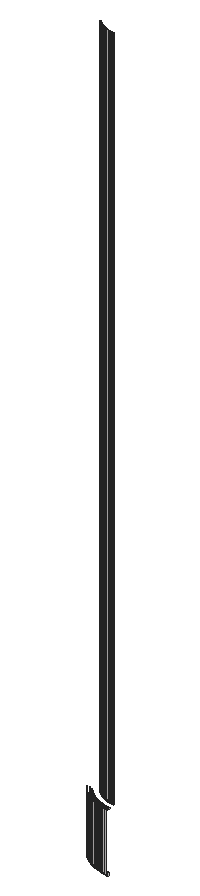
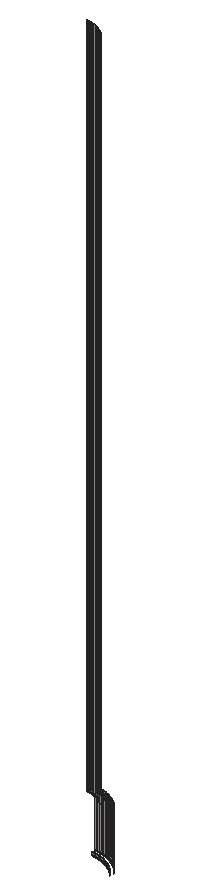
# SketchUp Ruby script. Lengths in inches.
U = 1.inch
M = Sketchup.active_model
def pt(a) = Geom::Point3d.new(a.map { |v| v * U })
def face(e, loops, mat)
  f = e.add_face(loops[0].map { |a| pt(a) })
  loops[1..].each { |l| e.add_face(l.map { |a| pt(a) }).erase! }
  f.material = f.back_material = mat if mat
  f
end
# faces: each face lists its corners as indices into pts; further lists are holes
def faces(e, pts, list, mat = nil) = list.each { |f| face(e, (f[0].is_a?(Array) ? f : [f]).map { |l| l.map { |i| pts[i] } }, mat) }
# xy, xz, yz: faces in a plane at the given z, y or x. An outline is a flat list of corners, or four numbers for a rectangle; further outlines are holes
def ring(l) = l.size == 4 ? [[l[0], l[1]], [l[2], l[1]], [l[2], l[3]], [l[0], l[3]]] : l.each_slice(2).to_a
def flat(e, list, mat, &to3) = list.each { |f| face(e, (f[0].is_a?(Array) ? f : [f]).map { |l| ring(l).map { |u, v| to3.(u, v) } }, mat) }
def xy(e, z, list, mat = nil) = flat(e, list, mat) { |x, y| [x, y, z] }
def xz(e, y, list, mat = nil) = flat(e, list, mat) { |x, z| [x, y, z] }
def yz(e, x, list, mat = nil) = flat(e, list, mat) { |y, z| [x, y, z] }
def lines(e, pts, list) = list.each { |a, b| e.add_line(pt(pts[a]), pt(pts[b])) }
# prism: a flat outline (further loops are holes) pulled along v
def prism(e, loops, v, mat = nil)
  f = face(e, loops, mat); d = Geom::Vector3d.new(v.map { |x| x * U })
  f.pushpull(f.normal.samedirection?(d) ? d.length : -d.length)
end
def box(e, o, s, mat = nil) = prism(e, [[o, [o[0] + s[0], o[1], o[2]], [o[0] + s[0], o[1] + s[1], o[2]], [o[0], o[1] + s[1], o[2]]]], [0, 0, s[2]], mat)
def at(x, y, z, deg = 0) = Geom::Transformation.translation(pt([x, y, z])) * Geom::Transformation.rotation(ORIGIN, Z_AXIS, deg.degrees)
def axes(o, x, y, z) = Geom::Transformation.new([*x, 0, *y, 0, *z, 0, *pt(o).to_a, 1])
def part(name) = M.definitions.add(name)
# library, detail: a bought-in or finely detailed component or shape, given as its bounding box
def library(name, o, s) = part(name).tap { |d| box(d.entities, o, s) }
def detail(e, o, s) = box(e.add_group.entities, o, s)
def put(e, d, t, mat = nil) = e.add_instance(d, t).tap { |i| i.material = mat if mat }
def group(e, t, mat = nil) = e.add_group.tap { |g| g.transformation = t; g.material = mat if mat }.entities
root = M.entities
M.materials.add("[Quartz Light Brown]").color = [215, 212, 212]
p = [[213.81,144.17,133],[213.81,144.17,132],[213.99,144.14,132],[213.99,144.14,133],[214.17,144.12,132],[214.17,144.12,133],
  [214.35,144.1,132],[214.35,144.1,133],[214.54,144.08,132],[214.54,144.08,133],[213.27,144.27,133],[213.27,144.27,132],
  [213.45,144.23,132],[213.45,144.23,133],[213.63,144.2,132],[213.63,144.2,133],[212.73,144.39,133],[212.73,144.39,132],
  [212.91,144.35,132],[212.91,144.35,133],[213.09,144.31,132],[213.09,144.31,133],[212.375,144.48,133],[212.375,144.48,132],
  [212.55,144.43,132],[212.55,144.43,133],[212.02,144.58,133],[212.02,144.58,132],[212.2,144.53,132],[212.2,144.53,133],
  [211.67,144.69,133],[211.67,144.69,132],[211.85,144.63,132],[211.85,144.63,133],[211.33,144.8,133],[211.33,144.8,132],
  [211.5,144.74,132],[211.5,144.74,133],[211.15,144.87,133],[211.15,144.87,132],[210.8125,145,133],[210.8125,145,132],
  [210.98,144.93,132],[210.98,144.93,133],[210.64,145.07,133],[210.64,145.07,132],[210.31,145.21,133],[210.31,145.21,132],
  [210.47,145.14,132],[210.47,145.14,133],[210.14,145.29,133],[210.14,145.29,132],[209.97,145.36,133],[209.97,145.36,132],
  [209.64,145.53,133],[209.64,145.53,132],[209.81,145.44,132],[209.81,145.44,133],[209.48,145.61,133],[209.48,145.61,132],
  [209.32,145.7,133],[209.32,145.7,132],[209.16,145.79,133],[209.16,145.79,132],[209,145.875,133],[209,145.875,132],
  [208.84,145.97,133],[208.84,145.97,132],[208.69,146.0625,133],[208.69,146.0625,132],[208.53,146.16,133],[208.53,146.16,132],
  [208.375,146.26,133],[208.375,146.26,132],[208.22,146.36,133],[208.22,146.36,132],[208.07,146.46,133],[208.07,146.46,132],
  [207.92,146.57,133],[207.92,146.57,132],[207.77,146.67,133],[207.77,146.67,132],[207.625,146.78,133],[207.625,146.78,132],
  [207.48,146.89,133],[207.48,146.89,132],[207.33,147.01,133],[207.33,147.01,132],[207.19,147.12,133],[207.19,147.12,132],
  [207.05,147.24,133],[207.05,147.24,132],[206.91,147.35,133],[206.91,147.35,132],[206.77,147.47,133],[206.77,147.47,132],
  [206.63,147.6,133],[206.63,147.6,132],[206.5,147.72,133],[206.5,147.72,132],[206.36,147.84,133],[206.36,147.84,132],
  [206.23,147.97,133],[206.23,147.97,132],[206.1,148.1,133],[206.1,148.1,132],[205.97,148.23,133],[205.97,148.23,132],
  [205.84,148.36,133],[205.84,148.36,132],[205.72,148.5,133],[205.72,148.5,132],[205.6,148.63,133],[205.6,148.63,132],
  [205.47,148.77,133],[205.47,148.77,132],[205.35,148.91,133],[205.35,148.91,132],[205.24,149.05,133],[205.24,149.05,132],
  [214.04,143.13,133],[214.04,143.13,150],[213.85,143.16,150],[213.85,143.16,133],[214.24,143.1,133],[214.24,143.1,150],
  [214.43,143.08,133],[214.43,143.08,150],[213.46,143.22,133],[213.46,143.22,150],[213.27,143.25,150],[213.27,143.25,133],
  [213.65,143.18,133],[213.65,143.18,150],[212.88,143.33,133],[212.88,143.33,150],[212.69,143.37,150],[212.69,143.37,133],
  [213.07,143.29,133],[213.07,143.29,150],[212.5,143.41,133],[212.5,143.41,150],[212.31,143.46,150],[212.31,143.46,133],
  [212.12,143.51,133],[212.12,143.51,150],[211.93,143.5625,150],[211.93,143.5625,133],[211.74,143.62,133],[211.74,143.62,150],
  [211.55,143.67,150],[211.55,143.67,133],[211.36,143.73,133],[211.36,143.73,150],[211.18,143.8,150],[211.18,143.8,133],
  [210.99,143.86,150],[210.99,143.86,133],[210.81,143.93,133],[210.81,143.93,150],[210.625,144,150],[210.625,144,133],
  [210.44,144.07,150],[210.44,144.07,133],[210.26,144.14,133],[210.26,144.14,150],[210.08,144.22,150],[210.08,144.22,133],
  [209.9,144.3,150],[209.9,144.3,133],[209.72,144.38,150],[209.72,144.38,133],[209.54,144.46,150],[209.54,144.46,133],
  [209.37,144.55,133],[209.37,144.55,150],[209.19,144.63,150],[209.19,144.63,133],[209.02,144.73,150],[209.02,144.73,133],
  [208.84,144.82,150],[208.84,144.82,133],[208.67,144.91,150],[208.67,144.91,133],[208.5,145.01,150],[208.5,145.01,133],
  [208.33,145.11,150],[208.33,145.11,133],[208.16,145.21,150],[208.16,145.21,133],[208,145.3125,150],[208,145.3125,133],
  [207.83,145.42,150],[207.83,145.42,133],[207.67,145.53,150],[207.67,145.53,133],[207.5,145.64,150],[207.5,145.64,133],
  [207.34,145.75,150],[207.34,145.75,133],[207.18,145.86,150],[207.18,145.86,133],[207.03,145.98,150],[207.03,145.98,133],
  [206.87,146.1,150],[206.87,146.1,133],[206.71,146.22,150],[206.71,146.22,133],[206.56,146.34,150],[206.56,146.34,133],
  [206.41,146.47,150],[206.41,146.47,133],[206.26,146.59,150],[206.26,146.59,133],[206.11,146.72,150],[206.11,146.72,133],
  [205.96,146.85,150],[205.96,146.85,133],[205.82,146.99,150],[205.82,146.99,133],[205.67,147.12,150],[205.67,147.12,133],
  [205.53,147.26,150],[205.53,147.26,133],[205.39,147.39,150],[205.39,147.39,133],[205.26,147.53,150],[205.26,147.53,133],
  [205.12,147.67,150],[205.12,147.67,133],[204.99,147.82,150],[204.99,147.82,133],[204.85,147.96,150],[204.85,147.96,133],
  [204.72,148.11,150],[204.72,148.11,133],[204.59,148.26,150],[204.59,148.26,133],[204.47,148.41,150],[204.47,148.41,133],
  [204.34,148.56,150],[204.34,148.56,133],[204.22,148.71,150],[204.22,148.71,133],[204.1,148.87,150],[204.1,148.87,133],
  [203.98,149.03,150],[203.98,149.03,133],[214.14,143.87,150],[214.33,143.85,150],[214.33,143.85,149.75],[214.14,143.87,149.75],
  [214.51,143.83,150],[214.51,143.83,149.75],[213.59,143.96,150],[213.77,143.93,150],[213.77,143.93,149.75],[213.59,143.96,149.75],
  [213.96,143.9,150],[213.96,143.9,149.75],[213.04,144.0625,150],[213.22,144.02,150],[213.22,144.02,149.75],[213.04,144.0625,149.75],
  [213.4,143.99,150],[213.4,143.99,149.75],[212.49,144.1875,150],[212.67,144.14,150],[212.67,144.14,149.75],[212.49,144.1875,149.75],
  [212.86,144.1,150],[212.86,144.1,149.75],[212.13,144.29,150],[212.3125,144.24,150],[212.3125,144.24,149.75],[212.13,144.29,149.75],
  [211.77,144.39,150],[211.95,144.34,150],[211.95,144.34,149.75],[211.77,144.39,149.75],[214.38,144.35,150],[214.21,144.37,150],
  [214.21,144.37,149.75],[214.38,144.35,149.75],[214.5625,144.33,150],[214.5625,144.33,149.75],[211.42,144.51,150],[211.6,144.45,150],
  [211.6,144.45,149.75],[211.42,144.51,149.75],[213.67,144.45,150],[213.49,144.48,150],[213.49,144.48,149.75],[213.67,144.45,149.75],
  [213.85,144.42,150],[213.85,144.42,149.75],[214.03,144.39,150],[214.03,144.39,149.75],[211.24,144.57,150],[211.24,144.57,149.75],
  [213.32,144.51,150],[213.14,144.55,150],[213.14,144.55,149.75],[213.32,144.51,149.75],[210.89,144.7,150],[211.07,144.63,150],
  [211.07,144.63,149.75],[210.89,144.7,149.75],[212.79,144.63,150],[212.62,144.67,150],[212.62,144.67,149.75],[212.79,144.63,149.75],
  [212.97,144.59,150],[212.97,144.59,149.75],[210.72,144.76,150],[210.72,144.76,149.75],[212.44,144.72,150],[212.27,144.77,150],
  [212.27,144.77,149.75],[212.44,144.72,149.75],[210.375,144.91,150],[210.55,144.83,150],[210.55,144.83,149.75],[210.375,144.91,149.75],
  [212.09,144.82,150],[211.92,144.87,150],[211.92,144.87,149.75],[212.09,144.82,149.75],[210.2,144.98,150],[210.2,144.98,149.75],
  [211.75,144.92,150],[211.58,144.98,150],[211.58,144.98,149.75],[211.75,144.92,149.75],[210.03,145.06,150],[210.03,145.06,149.75],
  [211.41,145.04,150],[211.24,145.1,150],[211.24,145.1,149.75],[211.41,145.04,149.75],[209.7,145.22,150],[209.87,145.14,150],
  [209.87,145.14,149.75],[209.7,145.22,149.75],[211.07,145.16,150],[211.07,145.16,149.75],[209.53,145.3,150],[209.53,145.3,149.75],
  [210.9,145.23,150],[210.74,145.3,150],[210.74,145.3,149.75],[210.9,145.23,149.75],[209.36,145.39,150],[209.36,145.39,149.75],
  [210.57,145.37,150],[210.57,145.37,149.75],[209.2,145.48,150],[209.2,145.48,149.75],[210.41,145.4375,150],[210.24,145.51,150],
  [210.24,145.51,149.75],[210.41,145.4375,149.75],[209.04,145.57,150],[209.04,145.57,149.75],[210.08,145.59,150],[210.08,145.59,149.75],
  [208.875,145.66,150],[208.875,145.66,149.75],[209.92,145.67,150],[209.92,145.67,149.75],[208.71,145.75,150],[208.71,145.75,149.75],
  [209.76,145.75,150],[209.6,145.83,150],[209.6,145.83,149.75],[209.76,145.75,149.75],[208.4,145.95,150],[208.55,145.85,150],
  [208.55,145.85,149.75],[208.4,145.95,149.75],[209.4375,145.92,150],[209.4375,145.92,149.75],[208.24,146.05,150],[208.24,146.05,149.75],
  [209.28,146,150],[209.28,146,149.75],[208.08,146.15,150],[208.08,146.15,149.75],[209.125,146.09,150],[209.125,146.09,149.75],
  [208.97,146.18,150],[208.97,146.18,149.75],[207.93,146.26,150],[207.93,146.26,149.75],[208.82,146.28,150],[208.82,146.28,149.75],
  [207.78,146.36,150],[207.78,146.36,149.75],[208.66,146.37,150],[208.66,146.37,149.75],[207.625,146.47,150],[207.625,146.47,149.75],
  [208.51,146.47,150],[208.51,146.47,149.75],[207.47,146.58,150],[207.47,146.58,149.75],[208.36,146.57,150],[208.36,146.57,149.75],
  [207.33,146.69,150],[207.33,146.69,149.75],[208.21,146.67,150],[208.21,146.67,149.75],[207.18,146.81,150],[207.18,146.81,149.75],
  [208.0625,146.77,150],[208.0625,146.77,149.75],[207.03,146.93,150],[207.03,146.93,149.75],[207.92,146.875,150],[207.92,146.875,149.75],
  [206.89,147.04,150],[206.89,147.04,149.75],[207.77,146.98,150],[207.77,146.98,149.75],[206.75,147.16,150],[206.75,147.16,149.75],
  [207.63,147.09,150],[207.63,147.09,149.75],[207.49,147.2,150],[207.49,147.2,149.75],[206.6,147.29,150],[206.6,147.29,149.75],
  [207.35,147.3125,150],[207.35,147.3125,149.75],[206.46,147.41,150],[206.46,147.41,149.75],[207.21,147.43,150],[207.21,147.43,149.75],
  [206.33,147.54,150],[206.33,147.54,149.75],[207.07,147.54,150],[207.07,147.54,149.75],[206.19,147.66,150],[206.19,147.66,149.75],
  [206.93,147.66,150],[206.93,147.66,149.75],[206.06,147.79,150],[206.06,147.79,149.75],[206.8,147.78,150],[206.8,147.78,149.75],
  [205.92,147.92,150],[205.92,147.92,149.75],[206.67,147.9,150],[206.67,147.9,149.75],[205.79,148.06,150],[205.79,148.06,149.75],
  [206.54,148.03,150],[206.54,148.03,149.75],[206.41,148.15,150],[206.41,148.15,149.75],[205.66,148.19,150],[205.66,148.19,149.75],
  [205.54,148.33,150],[205.54,148.33,149.75],[206.28,148.28,150],[206.28,148.28,149.75],[205.41,148.46,150],[205.41,148.46,149.75],
  [206.15,148.41,150],[206.15,148.41,149.75],[206.03,148.54,150],[206.03,148.54,149.75],[205.29,148.6,150],[205.29,148.6,149.75],
  [205.9,148.67,150],[205.9,148.67,149.75],[205.16,148.75,150],[205.16,148.75,149.75],[205.04,148.89,150],[205.04,148.89,149.75],
  [205.78,148.8,150],[205.78,148.8,149.75],[205.66,148.93,150],[205.66,148.93,149.75],[204.93,149.03,150],[204.93,149.03,149.75],
  [214.12,146.15,150],[214.12,146.15,354],[213.97,146.17,354],[213.97,146.17,150],[214.28,146.125,150],[214.28,146.125,354],
  [214.43,146.1,150],[214.43,146.1,354],[214.59,146.08,150],[214.59,146.08,354],[213.66,146.23,150],[213.66,146.23,354],
  [213.51,146.26,354],[213.51,146.26,150],[213.8125,146.2,150],[213.8125,146.2,354],[213.2,146.33,150],[213.2,146.33,354],
  [213.05,146.37,354],[213.05,146.37,150],[213.35,146.3,150],[213.35,146.3,354],[212.89,146.41,150],[212.89,146.41,354],
  [212.74,146.45,354],[212.74,146.45,150],[212.44,146.54,150],[212.44,146.54,354],[212.29,146.59,354],[212.29,146.59,150],
  [212.59,146.49,150],[212.59,146.49,354],[212.14,146.64,150],[212.14,146.64,354],[211.99,146.6875,354],[211.99,146.6875,150],
  [211.85,146.74,150],[211.85,146.74,354],[211.7,146.8,354],[211.7,146.8,150],[211.55,146.85,354],[211.55,146.85,150],
  [211.41,146.91,150],[211.41,146.91,354],[211.26,146.97,354],[211.26,146.97,150],[211.12,147.04,150],[211.12,147.04,354],
  [210.98,147.1,354],[210.98,147.1,150],[210.83,147.17,354],[210.83,147.17,150],[210.69,147.24,150],[210.69,147.24,354],
  [210.55,147.31,354],[210.55,147.31,150],[210.41,147.38,354],[210.41,147.38,150],[210.27,147.45,354],[210.27,147.45,150],
  [210.14,147.53,150],[210.14,147.53,354],[210,147.61,354],[210,147.61,150],[209.86,147.6875,354],[209.86,147.6875,150],
  [209.73,147.77,354],[209.73,147.77,150],[209.6,147.85,354],[209.6,147.85,150],[209.46,147.9375,150],[209.46,147.9375,354],
  [209.33,148.02,354],[209.33,148.02,150],[209.2,148.11,354],[209.2,148.11,150],[209.07,148.2,354],[209.07,148.2,150],
  [208.95,148.29,354],[208.95,148.29,150],[208.82,148.38,354],[208.82,148.38,150],[208.69,148.48,354],[208.69,148.48,150],
  [208.57,148.58,354],[208.57,148.58,150],[208.45,148.67,354],[208.45,148.67,150],[208.33,148.77,354],[208.33,148.77,150],
  [208.21,148.875,354],[208.21,148.875,150],[208.09,148.98,354],[208.09,148.98,150]]
faces(root,p,[[0,1,2,3],[3,2,4,5],[5,4,6,7],[7,6,8,9],[10,11,12,13],[13,12,14,15],[15,14,1,0],[16,17,18,19],
  [19,18,20,21],[21,20,11,10],[22,23,24,25],[25,24,17,16],[26,27,28,29],[29,28,23,22],[30,31,32,33],[33,32,27,26],
  [34,35,36,37],[37,36,31,30],[38,39,35,34],[40,41,42,43],[43,42,39,38],[44,45,41,40],[46,47,48,49],[49,48,45,44],
  [50,51,47,46],[52,53,51,50],[54,55,56,57],[57,56,53,52],[58,59,55,54],[60,61,59,58],[62,63,61,60],[64,65,63,62],
  [66,67,65,64],[68,69,67,66],[70,71,69,68],[72,73,71,70],[74,75,73,72],[76,77,75,74],[78,79,77,76],[80,81,79,78],
  [82,83,81,80],[84,85,83,82],[86,87,85,84],[88,89,87,86],[90,91,89,88],[92,93,91,90],[94,95,93,92],[96,97,95,94],
  [98,99,97,96],[100,101,99,98],[102,103,101,100],[104,105,103,102],[106,107,105,104],[108,109,107,106],[110,111,109,108],[112,113,111,110],
  [114,115,113,112],[116,117,115,114],[118,119,117,116],[120,121,122,123],[124,125,121,120],[126,127,125,124],[128,129,130,131],[132,133,129,128],
  [123,122,133,132],[134,135,136,137],[138,139,135,134],[131,130,139,138],[140,141,142,143],[137,136,141,140],[144,145,146,147],[143,142,145,144],
  [148,149,150,151],[147,146,149,148],[152,153,154,155],[151,150,153,152],[155,154,156,157],[158,159,160,161],[157,156,159,158],[161,160,162,163],
  [164,165,166,167],[163,162,165,164],[167,166,168,169],[169,168,170,171],[171,170,172,173],[174,175,176,177],[173,172,175,174],[177,176,178,179],
  [179,178,180,181],[181,180,182,183],[183,182,184,185],[185,184,186,187],[187,186,188,189],[189,188,190,191],[191,190,192,193],[193,192,194,195],
  [195,194,196,197],[197,196,198,199],[199,198,200,201],[201,200,202,203],[203,202,204,205],[205,204,206,207],[207,206,208,209],[209,208,210,211],
  [211,210,212,213],[213,212,214,215],[215,214,216,217],[217,216,218,219],[219,218,220,221],[221,220,222,223],[223,222,224,225],[225,224,226,227],
  [227,226,228,229],[229,228,230,231],[231,230,232,233],[233,232,234,235],[235,234,236,237],[237,236,238,239],[239,238,240,241],[241,240,242,243],
  [243,242,244,245],[245,244,246,247],[248,249,250,251],[249,252,253,250],[254,255,256,257],[255,258,259,256],[258,248,251,259],[260,261,262,263],
  [261,264,265,262],[264,254,257,265],[266,267,268,269],[267,270,271,268],[270,260,263,271],[272,273,274,275],[273,266,269,274],[276,277,278,279],
  [277,272,275,278],[280,281,282,283],[284,280,283,285],[286,287,288,289],[287,276,279,288],[290,291,292,293],[294,290,293,295],[296,294,295,297],
  [281,296,297,282],[298,286,289,299],[300,301,302,303],[291,300,303,292],[304,305,306,307],[305,298,299,306],[308,309,310,311],[312,308,311,313],
  [301,312,313,302],[314,304,307,315],[316,317,318,319],[309,316,319,310],[320,321,322,323],[321,314,315,322],[324,325,326,327],[317,324,327,318],
  [328,320,323,329],[330,331,332,333],[325,330,333,326],[334,328,329,335],[336,337,338,339],[331,336,339,332],[340,341,342,343],[341,334,335,342],
  [337,344,345,338],[346,340,343,347],[348,349,350,351],[344,348,351,345],[352,346,347,353],[349,354,355,350],[356,352,353,357],[358,359,360,361],
  [354,358,361,355],[362,356,357,363],[359,364,365,360],[366,362,363,367],[364,368,369,365],[370,366,367,371],[372,373,374,375],[368,372,375,369],
  [376,377,378,379],[377,370,371,378],[373,380,381,374],[382,376,379,383],[380,384,385,381],[386,382,383,387],[384,388,389,385],[388,390,391,389],
  [392,386,387,393],[390,394,395,391],[396,392,393,397],[394,398,399,395],[400,396,397,401],[398,402,403,399],[404,400,401,405],[402,406,407,403],
  [408,404,405,409],[406,410,411,407],[412,408,409,413],[410,414,415,411],[416,412,413,417],[414,418,419,415],[420,416,417,421],[418,422,423,419],
  [424,420,421,425],[422,426,427,423],[426,428,429,427],[430,424,425,431],[428,432,433,429],[434,430,431,435],[432,436,437,433],[438,434,435,439],
  [436,440,441,437],[442,438,439,443],[440,444,445,441],[446,442,443,447],[444,448,449,445],[450,446,447,451],[448,452,453,449],[454,450,451,455],
  [452,456,457,453],[456,458,459,457],[460,454,455,461],[462,460,461,463],[458,464,465,459],[466,462,463,467],[464,468,469,465],[468,470,471,469],
  [472,466,467,473],[470,474,475,471],[476,472,473,477],[478,476,477,479],[474,480,481,475],[480,482,483,481],[484,478,479,485],[486,487,488,489],
  [490,491,487,486],[492,493,491,490],[494,495,493,492],[496,497,498,499],[500,501,497,496],[489,488,501,500],[502,503,504,505],[506,507,503,502],
  [499,498,507,506],[508,509,510,511],[505,504,509,508],[512,513,514,515],[516,517,513,512],[511,510,517,516],[518,519,520,521],[515,514,519,518],
  [522,523,524,525],[521,520,523,522],[525,524,526,527],[528,529,530,531],[527,526,529,528],[532,533,534,535],[531,530,533,532],[535,534,536,537],
  [538,539,540,541],[537,536,539,538],[541,540,542,543],[543,542,544,545],[546,547,548,549],[545,544,547,546],[549,548,550,551],[551,550,552,553],
  [553,552,554,555],[556,557,558,559],[555,554,557,556],[559,558,560,561],[561,560,562,563],[563,562,564,565],[565,564,566,567],[567,566,568,569],
  [569,568,570,571],[571,570,572,573],[573,572,574,575],[575,574,576,577],[577,576,578,579]],"[Quartz Light Brown]")
